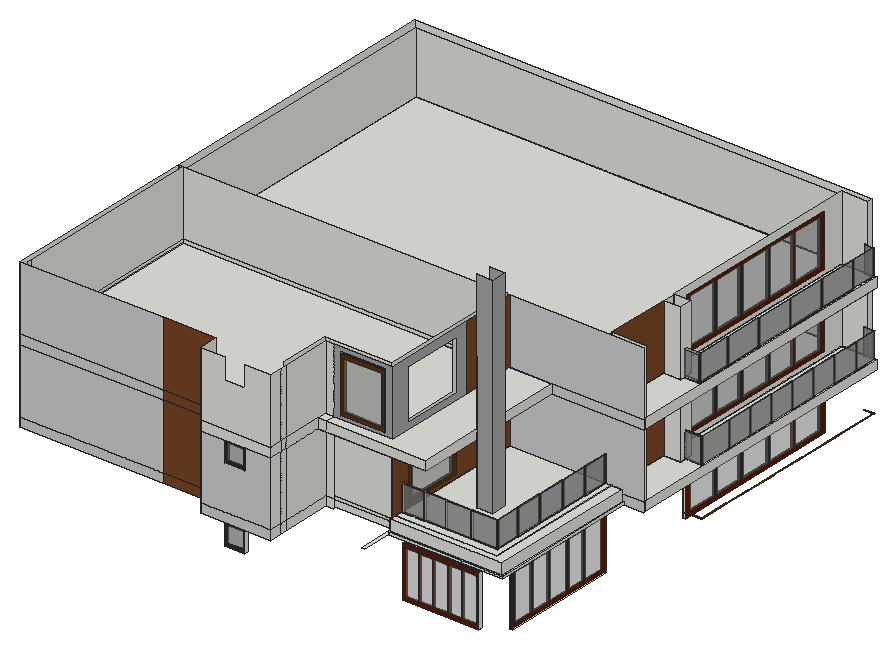
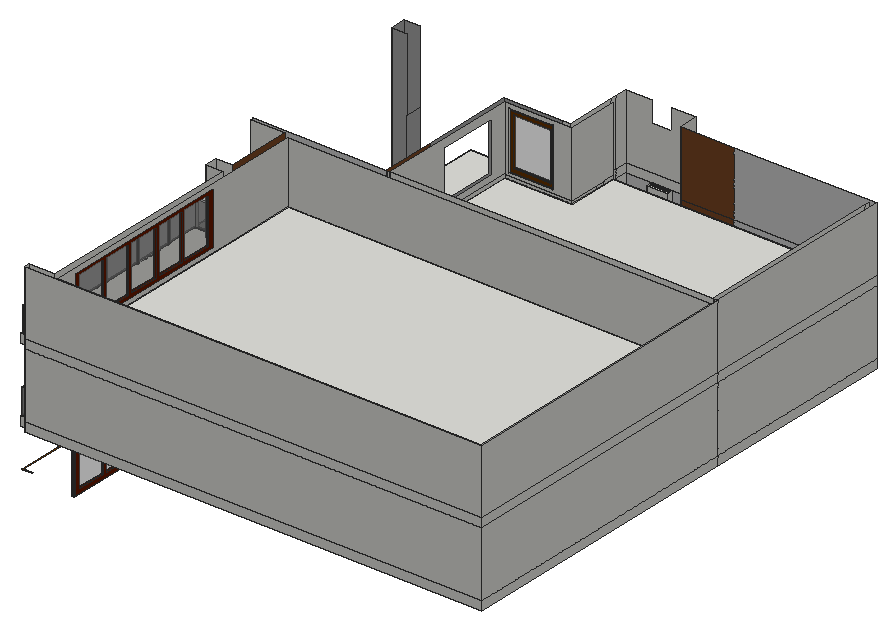
# SketchUp Ruby script. Lengths in inches.
U = 1.inch
M = Sketchup.active_model
def pt(a) = Geom::Point3d.new(a.map { |v| v * U })
def face(e, loops, mat)
  f = e.add_face(loops[0].map { |a| pt(a) })
  loops[1..].each { |l| e.add_face(l.map { |a| pt(a) }).erase! }
  f.material = f.back_material = mat if mat
  f
end
# faces: each face lists its corners as indices into pts; further lists are holes
def faces(e, pts, list, mat = nil) = list.each { |f| face(e, (f[0].is_a?(Array) ? f : [f]).map { |l| l.map { |i| pts[i] } }, mat) }
# xy, xz, yz: faces in a plane at the given z, y or x. An outline is a flat list of corners, or four numbers for a rectangle; further outlines are holes
def ring(l) = l.size == 4 ? [[l[0], l[1]], [l[2], l[1]], [l[2], l[3]], [l[0], l[3]]] : l.each_slice(2).to_a
def flat(e, list, mat, &to3) = list.each { |f| face(e, (f[0].is_a?(Array) ? f : [f]).map { |l| ring(l).map { |u, v| to3.(u, v) } }, mat) }
def xy(e, z, list, mat = nil) = flat(e, list, mat) { |x, y| [x, y, z] }
def xz(e, y, list, mat = nil) = flat(e, list, mat) { |x, z| [x, y, z] }
def yz(e, x, list, mat = nil) = flat(e, list, mat) { |y, z| [x, y, z] }
def lines(e, pts, list) = list.each { |a, b| e.add_line(pt(pts[a]), pt(pts[b])) }
# prism: a flat outline (further loops are holes) pulled along v
def prism(e, loops, v, mat = nil)
  f = face(e, loops, mat); d = Geom::Vector3d.new(v.map { |x| x * U })
  f.pushpull(f.normal.samedirection?(d) ? d.length : -d.length)
end
def box(e, o, s, mat = nil) = prism(e, [[o, [o[0] + s[0], o[1], o[2]], [o[0] + s[0], o[1] + s[1], o[2]], [o[0], o[1] + s[1], o[2]]]], [0, 0, s[2]], mat)
def at(x, y, z, deg = 0) = Geom::Transformation.translation(pt([x, y, z])) * Geom::Transformation.rotation(ORIGIN, Z_AXIS, deg.degrees)
def axes(o, x, y, z) = Geom::Transformation.new([*x, 0, *y, 0, *z, 0, *pt(o).to_a, 1])
def part(name) = M.definitions.add(name)
# library, detail: a bought-in or finely detailed component or shape, given as its bounding box
def library(name, o, s) = part(name).tap { |d| box(d.entities, o, s) }
def detail(e, o, s) = box(e.add_group.entities, o, s)
def put(e, d, t, mat = nil) = e.add_instance(d, t).tap { |i| i.material = mat if mat }
def group(e, t, mat = nil) = e.add_group.tap { |g| g.transformation = t; g.material = mat if mat }.entities
root = M.entities
M.materials.add("[Carrera Marble]").color = [207, 207, 207]
M.materials.add("[Color B08]").color = [102, 25, 0]
M.materials.add("[Color C08]").color = [102, 51, 0]
M.materials.add("[Stone Vein Gray]").color = [166, 165, 165]
M.materials.add("[Translucent Glass Gray]").color = [128, 128, 128]
M.materials["[Translucent Glass Gray]"].alpha = 0.5
M.materials.add("[Wood Veneer 01]").color = [120, 70, 37]
c1 = part("Group\#3")
xy(c1.entities,0,[[0,0,23.0625,440.625]],"[Color B08]")
xy(c1.entities,14.28,[[0,14.28,23.0625,92.65],[0,98.4,23.0625,173.71],[0,179.46,23.0625,261.65],[0,267.4,23.0625,340.59],[0,346.34,23.0625,426.35]],"[Color B08]")
xy(c1.entities,204.03,[[0,14.28,23.0625,92.65],[0,98.4,23.0625,173.71],[0,179.46,23.0625,261.65],[0,267.4,23.0625,340.59],[0,346.34,23.0625,426.35]],"[Color B08]")
xy(c1.entities,218.3125,[[0,0,23.0625,440.625]],"[Color B08]")
xz(c1.entities,0,[[0,0,23.0625,218.3125]],"[Color B08]")
xz(c1.entities,14.28,[[0,14.28,23.0625,204.03]],"[Color B08]")
xz(c1.entities,92.65,[[0,14.28,23.0625,204.03]],"[Color B08]")
xz(c1.entities,98.4,[[0,14.28,23.0625,204.03]],"[Color B08]")
xz(c1.entities,173.71,[[0,14.28,23.0625,204.03]],"[Color B08]")
xz(c1.entities,179.46,[[0,14.28,23.0625,204.03]],"[Color B08]")
xz(c1.entities,261.65,[[0,14.28,23.0625,204.03]],"[Color B08]")
xz(c1.entities,267.4,[[0,14.28,23.0625,204.03]],"[Color B08]")
xz(c1.entities,340.59,[[0,14.28,23.0625,204.03]],"[Color B08]")
xz(c1.entities,346.34,[[0,14.28,23.0625,204.03]],"[Color B08]")
xz(c1.entities,426.35,[[0,14.28,23.0625,204.03]],"[Color B08]")
xz(c1.entities,440.625,[[0,0,23.0625,218.3125]],"[Color B08]")
yz(c1.entities,0,[[[0,0,440.625,218.3125],[179.46,14.28,261.65,204.03],[346.34,14.28,426.35,204.03],[14.28,14.28,92.65,204.03],[98.4,14.28,173.71,204.03],[267.4,14.28,340.59,204.03]]],"[Color B08]")
yz(c1.entities,23.0625,[[[0,0,440.625,218.3125],[179.46,14.28,261.65,204.03],[346.34,14.28,426.35,204.03],[14.28,14.28,92.65,204.03],[98.4,14.28,173.71,204.03],[267.4,14.28,340.59,204.03]]],"[Color B08]")
yz(c1.entities,23.0625,[[14.28,14.28,92.65,204.03],[98.4,14.28,173.71,204.03],[179.46,14.28,261.65,204.03],[267.4,14.28,340.59,204.03],[346.34,14.28,426.35,204.03]],"[Translucent Glass Gray]")
c2 = part("Group\#1")
xy(c2.entities,0,[[0,0,21.625,260.4375]],"[Color C08]")
xy(c2.entities,20.42,[[0,20.42,21.625,240.02]],"[Color C08]")
xy(c2.entities,312.95,[[0,20.42,21.625,240.02]],"[Color C08]")
xy(c2.entities,333.375,[[0,0,21.625,260.4375]],"[Color C08]")
xz(c2.entities,0,[[0,0,21.625,333.375]],"[Color C08]")
xz(c2.entities,20.42,[[0,20.42,21.625,312.95]],"[Color C08]")
xz(c2.entities,240.02,[[0,20.42,21.625,312.95]],"[Color C08]")
xz(c2.entities,260.4375,[[0,0,21.625,333.375]],"[Color C08]")
yz(c2.entities,0,[[[0,0,260.4375,333.375],[20.42,20.42,240.02,312.95]]],"[Color C08]")
yz(c2.entities,21.625,[[[0,0,260.4375,333.375],[20.42,20.42,240.02,312.95]]],"[Color C08]")
yz(c2.entities,21.625,[[20.42,20.42,240.02,312.95]],"[Translucent Glass Gray]")
xy(root,290.68,[[791.375,750.16,797.375,1072.78]])
xy(root,291.2,[[801.71,337.86,807.71,553.05]])
xy(root,295.58,[[633.62,301.1875,774.31,308.3125]])
xy(root,329,[[828.5625,710.125,857.5,712.3125],[857.5,710.125,859.5,712.3125],[857.5,712.3125,859.5,769],[857.5,769,859.5,770.69],[857.5,770.69,859.5,819.125],
  [857.5,819.125,859.5,820.81],[857.5,820.81,859.5,876.0625],[857.5,876.0625,859.5,877.75],[857.5,877.75,859.5,943.6875],[857.5,943.6875,859.5,945.38],
  [857.5,945.38,859.5,1026.875],[857.5,1026.875,859.5,1028.56],[857.5,1028.56,859.5,1107.625],[841.07,1107.625,857.5,1109.875],[857.5,1107.625,859.5,1109.875]],"[Color C08]")
xy(root,362.75,[[406.64,171.6875,444.08,179.1875]])
xy(root,389.56,[[791.375,750.16,797.375,1072.78]])
xy(root,389.58,[[633.62,301.1875,774.31,308.3125]])
xy(root,390.2,[[801.71,337.86,807.71,553.05]])
xy(root,400.1875,[[406.64,171.6875,444.08,179.1875]])
xy(root,401,[[607.75,236.75,613.75,301.1875],[613.75,292.25,621.0625,308.3125],[621.0625,292.25,621.0625,301.1875,807.71,301.1875,807.71,573,824.77,573,824.77,292.25],[607.75,301.1875,613.75,308.3125],[621.0625,301.1875,621.0625,308.3125,801.71,308.3125,801.71,573,807.71,573,807.71,301.1875],
  [607.75,308.3125,613.75,573],[797.375,579,797.375,699.0625,828.5625,699.0625,828.5625,723.02,797.375,723.02,797.375,1111.6875,861.375,1111.6875,861.375,579]])
xy(root,405.375,[[613.75,292.25,824.77,295.8125],[821.21,295.8125,824.77,301.1875],[821.21,301.1875,824.77,573]])
xy(root,412,[[9,213.0625,9,573,607.75,573,607.75,308.3125,482.6875,308.3125,482.6875,213.0625],[613.75,308.3125,801.71,573],[9,579,791.375,1111.6875]])
xy(root,418,[[9,213.0625,482.6875,213.0625,482.6875,308.3125,607.75,308.3125,607.75,573,9,573],[9,579,791.375,1111.6875],[797.375,579,861.375,579,861.375,1111.6875,797.375,1111.6875,797.375,723.02,828.5625,723.02,828.5625,712.625,858.6875,712.625,858.6875,1109.5625,839.8,1109.5625,839.8,1110.6875,860.25,1110.6875,860.25,709.25,828.5625,709.25,828.5625,699.0625,797.375,699.0625],[828.5625,709.25,858.6875,712.625],[858.6875,709.25,860.25,712.625],
  [858.6875,712.625,860.25,773.63],[858.6875,773.63,860.25,774.72],[858.6875,774.72,860.25,822.32],[858.6875,822.32,860.25,823.4],[858.6875,823.4,860.25,871.01],
  [858.6875,871.01,860.25,872.09],[858.6875,872.09,860.25,919.69],[858.6875,919.69,860.25,920.78],[858.6875,920.78,860.25,968.38],[858.6875,968.38,860.25,969.47],
  [858.6875,969.47,860.25,1017.07],[858.6875,1017.07,860.25,1018.15],[858.6875,1018.15,860.25,1067.07],[858.6875,1067.07,860.25,1068.15],[858.6875,1068.15,858.6875,1109.5625,839.8,1109.5625,839.8,1110.6875,860.25,1110.6875,860.25,1068.15]])
xy(root,425.25,[[613.75,295.8125,821.21,295.8125,821.21,573,801.71,573,801.71,308.3125,613.75,308.3125],[613.75,308.3125,801.71,308.3125,801.71,573,791.71,573,791.71,322.5625,613.75,322.5625],[613.75,322.5625,616.79,324.5625],[616.79,322.5625,654.69,324.5625],[654.69,322.5625,656.21,324.5625],
  [656.21,322.5625,694.88,324.5625],[694.88,322.5625,696.39,324.5625],[696.39,322.5625,742.25,324.5625],[742.25,322.5625,743.77,324.5625],[743.77,322.5625,789.71,324.5625],
  [789.71,322.5625,791.71,324.5625],[[613.75,324.5625,789.71,573],[691.03,400.9,719.84,429.15]],[789.71,324.5625,791.71,369.72],[789.71,369.72,791.71,371.46],[789.71,371.46,791.71,420.78],
  [789.71,420.78,791.71,422.52],[789.71,422.52,791.71,473.28],[789.71,473.28,791.71,475.02],[789.71,475.02,791.71,524.28],[789.71,524.28,791.71,526.02],
  [789.71,526.02,791.71,569.45],[789.71,569.45,791.71,573]])
xy(root,425.87,[[791.375,750.16,797.375,1072.78]])
xy(root,430.3,[[607.75,336.9375,613.75,449.375]])
xy(root,466,[[828.5625,709.25,858.6875,712.625],[858.6875,709.25,860.25,712.625],[858.6875,712.625,860.25,773.63],[858.6875,773.63,860.25,774.72],[858.6875,774.72,860.25,822.32],
  [858.6875,822.32,860.25,823.4],[858.6875,823.4,860.25,871.01],[858.6875,871.01,860.25,872.09],[858.6875,872.09,860.25,919.69],[858.6875,919.69,860.25,920.78],
  [858.6875,920.78,860.25,968.38],[858.6875,968.38,860.25,969.47],[858.6875,969.47,860.25,1017.07],[858.6875,1017.07,860.25,1018.15],[858.6875,1018.15,860.25,1067.07],
  [858.6875,1067.07,860.25,1068.15],[858.6875,1068.15,860.25,1068.15,860.25,1110.6875,839.8,1110.6875,839.8,1109.5625,858.6875,1109.5625]],"[Color C08]")
xy(root,473.25,[[613.75,322.5625,616.79,324.5625],[616.79,322.5625,654.69,324.5625],[654.69,322.5625,656.21,324.5625],[656.21,322.5625,694.88,324.5625],[694.88,322.5625,696.39,324.5625],
  [696.39,322.5625,742.25,324.5625],[742.25,322.5625,743.77,324.5625],[743.77,322.5625,789.71,324.5625],[789.71,322.5625,791.71,324.5625],[789.71,324.5625,791.71,369.72],
  [789.71,369.72,791.71,371.46],[789.71,371.46,791.71,420.78],[789.71,420.78,791.71,422.52],[789.71,422.52,791.71,473.28],[789.71,473.28,791.71,475.02],
  [789.71,475.02,791.71,524.28],[789.71,524.28,791.71,526.02],[789.71,526.02,791.71,569.45],[789.71,569.45,791.71,573]],"[Color C08]")
xy(root,499.9375,[[406.64,171.6875,444.08,182.4375]])
xy(root,524.12,[[607.75,336.9375,613.75,449.375]])
xy(root,524.75,[[791.375,750.16,797.375,1072.78]])
xy(root,537.375,[[406.64,171.6875,444.08,182.4375]])
xy(root,538,[[491.3125,282.6875,506.0625,301.1875],[506.0625,282.6875,506.0625,301.1875,613.75,301.1875,613.75,573,691.03,573,691.03,282.6875],[797.375,579,797.375,699.0625,828.5625,699.0625,828.5625,723.02,797.375,723.02,797.375,1111.6875,861.375,1111.6875,861.375,579]])
xy(root,543,[[9,213.0625,9,573,607.75,573,607.75,308.3125,482.6875,308.3125,482.6875,213.0625]])
xy(root,549,[[9,213.0625,482.6875,213.0625,482.6875,308.3125,607.75,308.3125,607.75,573,9,573],[9,579,791.375,1111.6875]])
xy(root,555,[[491.3125,282.6875,506.0625,301.1875],[506.0625,282.6875,691.03,282.6875,691.03,573,613.75,573,613.75,301.1875,506.0625,301.1875],[9,579,791.375,1111.6875],[797.375,579,861.375,579,861.375,1111.6875,797.375,1111.6875,797.375,723.02,828.5625,723.02,828.5625,711.1875,856.375,711.1875,856.375,1110,841.51,1110,841.51,1110.8125,857.6875,1110.8125,857.6875,706.6875,828.5625,706.6875,828.5625,699.0625,797.375,699.0625],[828.5625,706.6875,856.375,711.1875],
  [856.375,706.6875,857.6875,711.1875],[856.375,711.1875,857.6875,772.08],[856.375,772.08,857.6875,773.74],[856.375,773.74,857.6875,844.71],[856.375,844.71,857.6875,846.37],
  [856.375,846.37,857.6875,917.33],[856.375,917.33,857.6875,918.99],[856.375,918.99,857.6875,989.96],[856.375,989.96,857.6875,991.62],[856.375,991.62,857.6875,1062.58],
  [856.375,1062.58,857.6875,1064.24],[856.375,1064.24,857.6875,1110],[841.51,1110,856.375,1110.8125],[856.375,1110,857.6875,1110.8125]])
xy(root,560.4,[[517.67,301.1875,599.79,308.3125]])
xy(root,562.5,[[791.375,750.16,797.375,1072.78]])
xz(root,171.6875,[[362.25,538,491.3125,555],[362.25,555,491.3125,555,491.3125,675.75,444.08,675.75,444.08,638.3125,406.64,638.3125,406.64,675.75,362.25,675.75]])
xz(root,171.6875,[[362.25,401,491.3125,418],[[362.25,418,491.3125,538],[406.64,499.9375,444.08,537.375]]],"[Carrera Marble]")
xz(root,179.1875,[[406.64,362.75,444.08,400.1875]])
xz(root,182.4375,[[406.64,499.9375,444.08,537.375]])
xz(root,207.0625,[[0,401,263.74,418],[0,418,263.74,538],[0,538,263.74,555],[0,555,263.74,675.75]],"[Carrera Marble]")
xz(root,207.0625,[[263.74,401,362.25,418],[263.74,418,362.25,538],[263.74,538,362.25,555],[263.74,555,362.25,675.75]],"[Wood Veneer 01]")
xz(root,213.0625,[[9,401,482.6875,412],[9,412,482.6875,418],[9,418,482.6875,543],[9,543,482.6875,549]])
xz(root,282.6875,[[491.3125,538,506.0625,555],[506.0625,538,691.03,555]])
xz(root,292.25,[[613.75,401,824.77,405.375]])
xz(root,295.8125,[[613.75,405.375,821.21,425.25]])
xz(root,301.1875,[[491.3125,401,506.0625,418],[491.3125,418,506.0625,538],[491.3125,555,506.0625,675.75]])
xz(root,301.1875,[[[506.0625,555,613.75,675.75],[517.67,560.4,599.79,667.78]]],"[Stone Vein Gray]")
xz(root,308.3125,[[482.6875,401,607.75,412],[613.75,401,801.71,405.375],[613.75,405.375,801.71,412],[482.6875,412,607.75,418],[613.75,412,801.71,425.25],
  [482.6875,418,607.75,538],[482.6875,538,607.75,543],[482.6875,543,607.75,549],[482.6875,549,607.75,555],[[482.6875,555,607.75,675.75],[517.67,560.4,599.79,667.78]]])
xz(root,322.5625,[[613.75,425.25,616.79,473.25],[654.69,425.25,656.21,473.25],[694.88,425.25,696.39,473.25],[742.25,425.25,743.77,473.25],[789.71,425.25,791.71,473.25]],"[Color C08]")
xz(root,322.5625,[[616.79,425.25,654.69,473.25],[656.21,425.25,694.88,473.25],[696.39,425.25,742.25,473.25],[743.77,425.25,789.71,473.25]],"[Translucent Glass Gray]")
xz(root,324.5625,[[654.69,425.25,656.21,473.25],[694.88,425.25,696.39,473.25],[742.25,425.25,743.77,473.25]])
xz(root,324.5625,[[616.79,425.25,654.69,473.25],[656.21,425.25,694.88,473.25],[696.39,425.25,742.25,473.25],[743.77,425.25,789.71,473.25]],"[Translucent Glass Gray]")
xz(root,336.9375,[[607.75,430.3,613.75,524.12]])
xz(root,337.86,[[801.71,291.2,807.71,390.2]])
xz(root,369.72,[[789.71,425.25,791.71,473.25]])
xz(root,371.46,[[789.71,425.25,791.71,473.25]])
xz(root,400.9,[[691.03,425.25,719.84,812]],"[Stone Vein Gray]")
xz(root,420.78,[[789.71,425.25,791.71,473.25]])
xz(root,422.52,[[789.71,425.25,791.71,473.25]])
xz(root,429.15,[[691.03,425.25,719.84,812]],"[Stone Vein Gray]")
xz(root,449.375,[[607.75,430.3,613.75,524.12]])
xz(root,473.28,[[789.71,425.25,791.71,473.25]])
xz(root,475.02,[[789.71,425.25,791.71,473.25]])
xz(root,524.28,[[789.71,425.25,791.71,473.25]])
xz(root,526.02,[[789.71,425.25,791.71,473.25]])
xz(root,553.05,[[801.71,291.2,807.71,390.2]])
xz(root,569.45,[[789.71,425.25,791.71,473.25]])
xz(root,573,[[0,401,9,418],[9,401,607.75,412],[607.75,401,613.75,418],[613.75,401,801.71,412],[801.71,401,824.77,405.375],
  [801.71,405.375,821.21,425.25],[9,412,607.75,418],[613.75,412,801.71,425.25],[0,418,9,538],[9,418,607.75,538],
  [607.75,418,613.75,538],[789.71,425.25,791.71,473.25],[0,538,9,555],[9,538,607.75,543],[607.75,538,691.03,555],
  [9,543,607.75,549],[9,549,607.75,555],[0,555,9,675],[9,555,607.75,675],[607.75,555,613.75,675]])
xz(root,573,[[824.77,401,861.375,401,861.375,418,821.21,418,821.21,405.375,824.77,405.375],[821.21,418,861.375,418,861.375,538,613.75,538,613.75,425.25,789.71,425.25,789.71,473.25,791.71,473.25,791.71,425.25,821.21,425.25],[691.03,538,861.375,555],[613.75,555,861.375,675]],"[Carrera Marble]")
xz(root,579,[[9,401,791.375,412],[797.375,401,861.375,418],[9,412,791.375,418],[9,418,791.375,538],[797.375,418,861.375,538],
  [9,538,791.375,549],[797.375,538,861.375,555],[9,549,791.375,555],[9,555,791.375,669],[797.375,555,861.375,675]])
xz(root,699.0625,[[797.375,401,828.5625,418],[797.375,418,828.5625,538],[797.375,538,828.5625,555],[797.375,555,828.5625,675]])
xz(root,706.6875,[[856.375,555,857.6875,603]],"[Color C08]")
xz(root,706.6875,[[828.5625,555,856.375,603]],"[Translucent Glass Gray]")
xz(root,709.25,[[858.6875,418,860.25,466]],"[Color C08]")
xz(root,709.25,[[828.5625,418,858.6875,466]],"[Translucent Glass Gray]")
xz(root,711.1875,[[856.375,555,857.6875,603]])
xz(root,711.1875,[[828.5625,555,856.375,603]],"[Translucent Glass Gray]")
xz(root,712.625,[[858.6875,418,860.25,466]])
xz(root,712.625,[[828.5625,418,858.6875,466]],"[Translucent Glass Gray]")
xz(root,723.02,[[797.375,401,828.5625,418],[797.375,418,828.5625,538],[797.375,538,828.5625,555],[797.375,555,828.5625,675]])
xz(root,750.16,[[791.375,290.68,797.375,389.56],[791.375,425.87,797.375,524.75],[791.375,562.5,797.375,661.37]])
xz(root,772.08,[[856.375,555,857.6875,603]])
xz(root,773.63,[[858.6875,418,860.25,466]])
xz(root,773.74,[[856.375,555,857.6875,603]])
xz(root,774.72,[[858.6875,418,860.25,466]])
xz(root,822.32,[[858.6875,418,860.25,466]])
xz(root,823.4,[[858.6875,418,860.25,466]])
xz(root,844.71,[[856.375,555,857.6875,603]])
xz(root,846.37,[[856.375,555,857.6875,603]])
xz(root,871.01,[[858.6875,418,860.25,466]])
xz(root,872.09,[[858.6875,418,860.25,466]])
xz(root,917.33,[[856.375,555,857.6875,603]])
xz(root,918.99,[[856.375,555,857.6875,603]])
xz(root,919.69,[[858.6875,418,860.25,466]])
xz(root,920.78,[[858.6875,418,860.25,466]])
xz(root,968.38,[[858.6875,418,860.25,466]])
xz(root,969.47,[[858.6875,418,860.25,466]])
xz(root,989.96,[[856.375,555,857.6875,603]])
xz(root,991.62,[[856.375,555,857.6875,603]])
xz(root,1017.07,[[858.6875,418,860.25,466]])
xz(root,1018.15,[[858.6875,418,860.25,466]])
xz(root,1062.58,[[856.375,555,857.6875,603]])
xz(root,1064.24,[[856.375,555,857.6875,603]])
xz(root,1067.07,[[858.6875,418,860.25,466]])
xz(root,1068.15,[[858.6875,418,860.25,466]])
xz(root,1072.78,[[791.375,290.68,797.375,389.56],[791.375,425.87,797.375,524.75],[791.375,562.5,797.375,661.37]])
xz(root,1109.5625,[[839.8,418,858.6875,466]],"[Translucent Glass Gray]")
xz(root,1110,[[856.375,555,857.6875,603]])
xz(root,1110,[[841.51,555,856.375,603]],"[Translucent Glass Gray]")
xz(root,1110.6875,[[839.8,418,860.25,466]],"[Translucent Glass Gray]")
xz(root,1110.8125,[[856.375,555,857.6875,603]],"[Color C08]")
xz(root,1110.8125,[[841.51,555,856.375,603]],"[Translucent Glass Gray]")
xz(root,1111.6875,[[9,401,791.375,412],[797.375,401,845.0625,418],[845.0625,401,861.375,418],[9,412,791.375,418],[9,418,791.375,538],
  [797.375,418,845.0625,538],[9,538,791.375,549],[797.375,538,845.0625,555],[845.0625,538,861.375,555],[9,549,791.375,555],
  [9,555,791.375,669],[797.375,555,845.0625,675]])
xz(root,1120.6875,[[0,401,845.0625,418],[0,418,845.0625,538],[0,538,845.0625,555],[0,555,845.0625,675]])
yz(root,0,[[207.0625,401,573,418],[573,401,1120.6875,418],[207.0625,418,573,538],[573,418,1120.6875,538],[207.0625,538,573,555],
  [573,538,1120.6875,555],[207.0625,555,573,675.75],[573,555,1120.6875,675]])
yz(root,9,[[213.0625,401,222,412],[222,401,573,412],[579,401,1111.6875,412],[213.0625,412,222,418],[222,412,573,418],
  [579,412,1111.6875,418],[213.0625,418,222,538],[222,418,573,538],[579,418,1111.6875,538],[213.0625,538,222,543],
  [222,538,573,543],[579,538,1111.6875,549],[213.0625,543,222,549],[222,543,573,549],[213.0625,549,222,555],
  [222,549,573,555],[579,549,1111.6875,555],[213.0625,555,222,675.75],[222,555,573,675.75],[579,555,1111.6875,669]])
yz(root,362.25,[[171.6875,538,207.0625,555],[171.6875,555,207.0625,675.75]])
yz(root,362.25,[[171.6875,401,207.0625,418],[171.6875,418,207.0625,538]],"[Carrera Marble]")
yz(root,406.64,[[171.6875,362.75,179.1875,400.1875],[171.6875,499.9375,182.4375,537.375]])
yz(root,444.08,[[171.6875,362.75,179.1875,400.1875],[171.6875,499.9375,182.4375,537.375]])
yz(root,482.6875,[[213.0625,401,308.3125,412],[213.0625,412,242.8125,418],[242.8125,412,260.6875,418],[260.6875,412,308.3125,418],[213.0625,418,308.3125,538],
  [213.0625,538,308.3125,543],[213.0625,543,234.8,549],[234.8,543,253.3,549],[253.3,543,308.3125,549],[213.0625,549,234.8,555],
  [234.8,549,253.3,555],[253.3,549,308.3125,555],[213.0625,555,308.3125,675.75]])
yz(root,491.3125,[[171.6875,401,195.6875,418],[195.6875,401,207.0625,418],[207.0625,401,301.1875,418],[171.6875,418,195.6875,538],[195.6875,418,207.0625,538],
  [207.0625,418,301.1875,538],[171.6875,538,195.6875,555],[195.6875,538,207.0625,555],[207.0625,538,282.6875,555],[171.6875,555,195.6875,675.75],
  [195.6875,555,207.0625,675.75],[207.0625,555,301.1875,675.75]])
yz(root,517.67,[[301.1875,560.4,308.3125,667.78]])
yz(root,599.79,[[301.1875,560.4,308.3125,667.78]])
yz(root,607.75,[[308.3125,401,573,412],[308.3125,412,573,418],[[308.3125,418,573,538],[336.9375,430.3,449.375,524.12]],[308.3125,538,573,543],[308.3125,543,573,549],
  [308.3125,549,573,555],[[308.3125,555,573,675.75],[336.9375,566.18,449.375,659.99]]])
yz(root,613.75,[[292.25,401,292.25,405.375,295.8125,405.375,295.8125,425.25,301.1875,425.25,301.1875,401],[308.3125,401,573,412],[301.1875,405.375,308.3125,418],[308.3125,412,318.6875,418],[318.6875,412,573,418],
  [301.1875,418,308.3125,425.25],[308.3125,418,318.6875,425.25],[318.6875,418,573,425.25],[322.5625,425.25,324.5625,473.25]])
yz(root,613.75,[[[301.1875,555,472.61,675.75],[336.9375,566.18,449.375,659.99]]],"[Stone Vein Gray]")
yz(root,613.75,[[[301.1875,425.25,322.5625,425.25,322.5625,473.25,324.5625,473.25,324.5625,425.25,573,425.25,573,538,301.1875,538],[336.9375,430.3,449.375,524.12]],[472.61,555,573,675.75]],"[Wood Veneer 01]")
yz(root,616.79,[[322.5625,425.25,324.5625,473.25]])
yz(root,633.62,[[301.1875,295.58,308.3125,389.58]])
yz(root,654.69,[[322.5625,425.25,324.5625,473.25]])
yz(root,656.21,[[322.5625,425.25,324.5625,473.25]])
yz(root,691.03,[[400.9,425.25,429.15,538],[282.6875,538,400.9,555],[400.9,538,429.15,555],[429.15,538,573,555]])
yz(root,691.03,[[400.9,555,429.15,675.75]],"[Stone Vein Gray]")
yz(root,694.88,[[322.5625,425.25,324.5625,473.25]])
yz(root,696.39,[[322.5625,425.25,324.5625,473.25]])
yz(root,719.84,[[400.9,425.25,429.15,812]],"[Stone Vein Gray]")
yz(root,742.25,[[322.5625,425.25,324.5625,473.25]])
yz(root,743.77,[[322.5625,425.25,324.5625,473.25]])
yz(root,774.31,[[301.1875,295.58,308.3125,389.58]])
yz(root,789.71,[[322.5625,425.25,324.5625,473.25]])
yz(root,789.71,[[369.72,425.25,371.46,473.25],[420.78,425.25,422.52,473.25],[473.28,425.25,475.02,473.25],[524.28,425.25,526.02,473.25],[569.45,425.25,573,473.25]],"[Color C08]")
yz(root,789.71,[[324.5625,425.25,369.72,473.25],[371.46,425.25,420.78,473.25],[422.52,425.25,473.28,473.25],[475.02,425.25,524.28,473.25],[526.02,425.25,569.45,473.25]],"[Translucent Glass Gray]")
yz(root,791.375,[[579,401,1111.6875,412],[579,412,722.51,418],[722.51,412,729.83,418],[729.83,412,1111.6875,418],[[579,418,1111.6875,538],[750.16,425.87,1072.78,524.75]],
  [579,538,1111.6875,549],[579,549,740.34,555],[740.34,549,744.4,555],[744.4,549,1111.6875,555],[[579,555,1111.6875,669],[750.16,562.5,1072.78,661.37]]])
yz(root,791.71,[[322.5625,425.25,324.5625,473.25],[369.72,425.25,371.46,473.25],[420.78,425.25,422.52,473.25],[473.28,425.25,475.02,473.25],[524.28,425.25,526.02,473.25],
  [569.45,425.25,573,473.25]],"[Color C08]")
yz(root,791.71,[[324.5625,425.25,369.72,473.25],[371.46,425.25,420.78,473.25],[422.52,425.25,473.28,473.25],[475.02,425.25,524.28,473.25],[526.02,425.25,569.45,473.25]],"[Translucent Glass Gray]")
yz(root,797.375,[[579,401,699.0625,418],[723.02,401,1111.6875,418],[[723.02,418,1111.6875,538],[750.16,425.87,1072.78,524.75]],[579,538,699.0625,555],[723.02,538,1111.6875,555],
  [[723.02,555,1111.6875,675],[750.16,562.5,1072.78,661.37]]])
yz(root,797.375,[[579,418,699.0625,538],[579,555,699.0625,675]],"[Wood Veneer 01]")
yz(root,801.71,[[308.3125,401,573,405.375],[308.3125,405.375,573,412],[308.3125,412,573,425.25]])
yz(root,821.21,[[295.8125,405.375,573,425.25]])
yz(root,824.77,[[292.25,401,573,405.375]])
yz(root,828.5625,[[699.0625,401,723.02,418],[699.0625,418,709.25,418,709.25,466,712.625,466,712.625,418,723.02,418,723.02,538,699.0625,538],[709.25,418,712.625,466],[699.0625,538,723.02,555],[699.0625,555,706.6875,555,706.6875,603,711.1875,603,711.1875,555,723.02,555,723.02,675,699.0625,675],
  [706.6875,555,711.1875,603]])
yz(root,839.8,[[1109.5625,418,1110.6875,466]])
yz(root,841.51,[[1110,555,1110.8125,603]])
yz(root,845.0625,[[1111.6875,401,1120.6875,418],[1111.6875,418,1120.6875,538],[1111.6875,538,1120.6875,555],[1111.6875,555,1120.6875,675]])
yz(root,856.375,[[706.6875,555,711.1875,603],[1110,555,1110.8125,603]])
yz(root,856.375,[[772.08,555,773.74,603],[844.71,555,846.37,603],[917.33,555,918.99,603],[989.96,555,991.62,603],[1062.58,555,1064.24,603]],"[Color C08]")
yz(root,856.375,[[711.1875,555,772.08,603],[773.74,555,844.71,603],[846.37,555,917.33,603],[918.99,555,989.96,603],[991.62,555,1062.58,603],
  [1064.24,555,1110,603]],"[Translucent Glass Gray]")
yz(root,857.6875,[[706.6875,555,711.1875,603],[772.08,555,773.74,603],[844.71,555,846.37,603],[917.33,555,918.99,603],[989.96,555,991.62,603],
  [1062.58,555,1064.24,603],[1110,555,1110.8125,603]],"[Color C08]")
yz(root,857.6875,[[711.1875,555,772.08,603],[773.74,555,844.71,603],[846.37,555,917.33,603],[918.99,555,989.96,603],[991.62,555,1062.58,603],
  [1064.24,555,1110,603]],"[Translucent Glass Gray]")
yz(root,858.6875,[[709.25,418,712.625,466]])
yz(root,858.6875,[[773.63,418,774.72,466],[822.32,418,823.4,466],[871.01,418,872.09,466],[919.69,418,920.78,466],[968.38,418,969.47,466],
  [1017.07,418,1018.15,466],[1067.07,418,1068.15,466]],"[Color C08]")
yz(root,858.6875,[[712.625,418,773.63,466],[774.72,418,822.32,466],[823.4,418,871.01,466],[872.09,418,919.69,466],[920.78,418,968.38,466],
  [969.47,418,1017.07,466],[1018.15,418,1067.07,466],[1068.15,418,1109.5625,466]],"[Translucent Glass Gray]")
yz(root,860.25,[[709.25,418,712.625,466],[773.63,418,774.72,466],[822.32,418,823.4,466],[871.01,418,872.09,466],[919.69,418,920.78,466],
  [968.38,418,969.47,466],[1017.07,418,1018.15,466],[1067.07,418,1068.15,466]],"[Color C08]")
yz(root,860.25,[[712.625,418,773.63,466],[774.72,418,822.32,466],[823.4,418,871.01,466],[872.09,418,919.69,466],[920.78,418,968.38,466],
  [969.47,418,1017.07,466],[1018.15,418,1067.07,466],[1068.15,418,1110.6875,466]],"[Translucent Glass Gray]")
yz(root,861.375,[[579,401,1111.6875,418],[579,538,1111.6875,555]])
put(root,c1,axes([792.53,750.55,290.68],[0.21,0,0],[0,0.7313,0],[0,0,0.45291]))
put(root,c1,axes([802.87,337.86,291.2],[0.126,0,0],[0,0.48837,0],[0,0,0.45348]))
put(root,c1,axes([633.62,303.92,295.58],[0,-0.11844,0],[0.31929,0,0],[0,0,0.43058]))
put(root,c2,axes([406.64,173.97,362.75],[0,0.11448,0],[0.14375,0,0],[0,0,0.1123]))
put(root,c1,axes([792.53,750.55,425.87],[0.21,0,0],[0,0.7313,0],[0,0,0.45291]),"[Color C08]")
put(root,c2,axes([607.64,336.9375,430.3],[0.28,0,0],[0,0.43173,0],[0,0,0.28]))
put(root,c2,axes([406.64,173.97,499.9375],[0,0.11448,0],[0.14375,0,0],[0,0,0.1123]))
put(root,c2,axes([517.48,304.76,560.4],[0,-0.1652,0],[0.31605,0,0],[0,0,0.30934]))
put(root,c1,axes([792.53,750.55,562.5],[0.21,0,0],[0,0.7313,0],[0,0,0.45291]))
